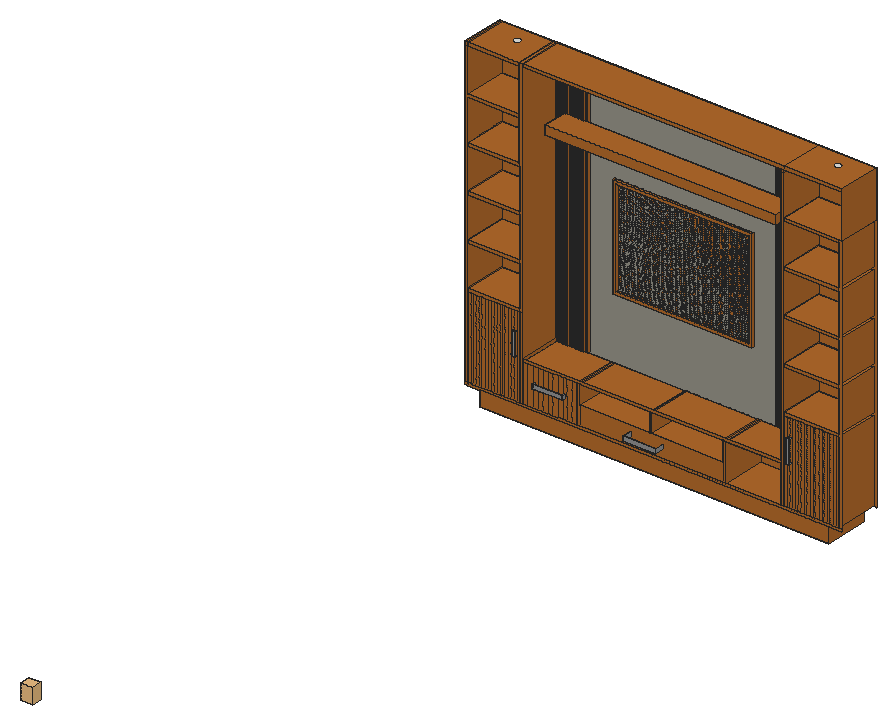
# SketchUp Ruby script. Lengths in millimetres.
U = 1.mm
M = Sketchup.active_model
def pt(a) = Geom::Point3d.new(a.map { |v| v * U })
def face(e, loops, mat)
  f = e.add_face(loops[0].map { |a| pt(a) })
  loops[1..].each { |l| e.add_face(l.map { |a| pt(a) }).erase! }
  f.material = f.back_material = mat if mat
  f
end
# faces: each face lists its corners as indices into pts; further lists are holes
def faces(e, pts, list, mat = nil) = list.each { |f| face(e, (f[0].is_a?(Array) ? f : [f]).map { |l| l.map { |i| pts[i] } }, mat) }
# xy, xz, yz: faces in a plane at the given z, y or x. An outline is a flat list of corners, or four numbers for a rectangle; further outlines are holes
def ring(l) = l.size == 4 ? [[l[0], l[1]], [l[2], l[1]], [l[2], l[3]], [l[0], l[3]]] : l.each_slice(2).to_a
def flat(e, list, mat, &to3) = list.each { |f| face(e, (f[0].is_a?(Array) ? f : [f]).map { |l| ring(l).map { |u, v| to3.(u, v) } }, mat) }
def xy(e, z, list, mat = nil) = flat(e, list, mat) { |x, y| [x, y, z] }
def xz(e, y, list, mat = nil) = flat(e, list, mat) { |x, z| [x, y, z] }
def yz(e, x, list, mat = nil) = flat(e, list, mat) { |y, z| [x, y, z] }
def lines(e, pts, list) = list.each { |a, b| e.add_line(pt(pts[a]), pt(pts[b])) }
# prism: a flat outline (further loops are holes) pulled along v
def prism(e, loops, v, mat = nil)
  f = face(e, loops, mat); d = Geom::Vector3d.new(v.map { |x| x * U })
  f.pushpull(f.normal.samedirection?(d) ? d.length : -d.length)
end
def box(e, o, s, mat = nil) = prism(e, [[o, [o[0] + s[0], o[1], o[2]], [o[0] + s[0], o[1] + s[1], o[2]], [o[0], o[1] + s[1], o[2]]]], [0, 0, s[2]], mat)
def at(x, y, z, deg = 0) = Geom::Transformation.translation(pt([x, y, z])) * Geom::Transformation.rotation(ORIGIN, Z_AXIS, deg.degrees)
def axes(o, x, y, z) = Geom::Transformation.new([*x, 0, *y, 0, *z, 0, *pt(o).to_a, 1])
def part(name) = M.definitions.add(name)
# library, detail: a bought-in or finely detailed component or shape, given as its bounding box
def library(name, o, s) = part(name).tap { |d| box(d.entities, o, s) }
def detail(e, o, s) = box(e.add_group.entities, o, s)
def put(e, d, t, mat = nil) = e.add_instance(d, t).tap { |i| i.material = mat if mat }
def group(e, t, mat = nil) = e.add_group.tap { |g| g.transformation = t; g.material = mat if mat }.entities
root = M.entities
M.materials.add("[Formica Graystone]").color = [149, 146, 135]
M.materials.add("[Metal Embossed]").color = [144, 144, 144]
M.materials.add("[Metal Rough]").color = [153, 157, 160]
M.materials.add("[Wood Bamboo]").color = [177, 105, 43]
c1 = library("Group145\#1",[149.2,164.2,242.8],[528.4,257.1,288.5])
xy(root,2329.8,[[2393.4,174.9,2398.1,175.5,2402.4,177.3,2406.2,180.1,2409,183.9,2410.8,188.2,2411.4,192.9,2410.8,197.5,2409,201.9,2406.2,205.6,2402.4,208.5,2398.1,210.3,2393.4,210.9,2388.8,210.3,2384.4,208.5,2380.7,205.6,2377.8,201.9,2376,197.5,2375.4,192.9,2376,188.2,2377.8,183.9,2380.7,180.1,2384.4,177.3,2388.8,175.5],[246.3,208.1,251.5,208.8,256.3,210.8,260.5,213.9,263.7,218.1,265.7,222.9,266.4,228.1,265.7,233.2,263.7,238.1,260.6,242.2,256.5,245.4,251.6,247.4,246.5,248.1,241.3,247.5,236.5,245.5,232.3,242.3,229.1,238.2,227.1,233.4,226.4,228.2,227,223,229,218.2,232.2,214.1,236.3,210.9,241.1,208.8]])
xy(root,2629.8,[[231.5,187.1,236.1,187.7,240.5,189.5,244.2,192.3,247.1,196.1,248.9,200.4,249.5,205.1,248.9,209.7,247.1,214.1,244.2,217.8,240.5,220.6,236.1,222.4,231.5,223.1,226.8,222.4,222.5,220.6,218.7,217.8,215.9,214.1,214.1,209.7,213.5,205.1,214.1,200.4,215.9,196.1,218.7,192.3,222.5,189.5,226.8,187.7],[2395.6,206.5,2400.2,206.8,2404.7,208.2,2408.7,210.7,2411.8,214.2,2414,218.4,2415,223,2414.8,227.7,2413.3,232.1,2410.8,236.1,2407.3,239.3,2403.1,241.4,2398.5,242.4,2393.9,242.2,2389.4,240.7,2385.4,238.2,2382.3,234.7,2380.1,230.6,2379.1,226,2379.3,221.3,2380.8,216.8,2383.3,212.8,2386.8,209.7,2391,207.5]])
xy(root,2929.8,[[244.8,192,249.5,192.4,253.9,193.9,257.8,196.6,260.9,200.1,262.9,204.4,263.8,209,263.4,213.7,261.9,218.1,259.2,222,255.7,225,251.4,227.1,246.8,228,242.1,227.6,237.7,226.1,233.8,223.4,230.8,219.8,228.7,215.6,227.8,211,228.2,206.3,229.7,201.9,232.4,198,236,194.9,240.2,192.9],[2398.3,207.7,2403,208.3,2407.3,210.1,2411.1,213,2413.9,216.7,2415.7,221,2416.3,225.7,2415.7,230.4,2413.9,234.7,2411.1,238.4,2407.3,241.3,2403,243.1,2398.3,243.7,2393.7,243.1,2389.3,241.3,2385.6,238.4,2382.8,234.7,2381,230.4,2380.3,225.7,2381,221,2382.8,216.7,2385.6,213,2389.3,210.1,2393.7,208.3]])
xy(root,3118.8,[[1326.6,220.4,1331.8,221.1,1336.6,223.1,1340.8,226.3,1344,230.4,1346,235.2,1346.6,240.4,1346,245.6,1344,250.4,1340.8,254.6,1336.6,257.7,1331.8,259.7,1326.6,260.4,1321.5,259.7,1316.6,257.7,1312.5,254.6,1309.3,250.4,1307.3,245.6,1306.6,240.4,1307.3,235.2,1309.3,230.4,1312.5,226.3,1316.6,223.1,1321.5,221.1],[779,222.1,784.2,222.8,789,224.8,793.1,228,796.3,232.1,798.3,236.9,799,242.1,798.3,247.3,796.3,252.1,793.1,256.3,789,259.4,784.2,261.4,779,262.1,773.8,261.4,769,259.4,764.8,256.3,761.7,252.1,759.7,247.3,759,242.1,759.7,236.9,761.7,232.1,764.8,228,769,224.8,773.8,222.8],[1912.4,226.4,1917.6,227.1,1922.4,229.1,1926.6,232.3,1929.7,236.4,1931.7,241.2,1932.4,246.4,1931.7,251.6,1929.7,256.4,1926.6,260.6,1922.4,263.7,1917.6,265.7,1912.4,266.4,1907.2,265.7,1902.4,263.7,1898.3,260.6,1895.1,256.4,1893.1,251.6,1892.4,246.4,1893.1,241.2,1895.1,236.4,1898.3,232.3,1902.4,229.1,1907.2,227.1]])
xy(root,3229.8,[[223.6,166.8,228.3,167.4,232.6,169.2,236.3,172.1,239.2,175.8,241,180.2,241.6,184.8,241,189.5,239.2,193.8,236.3,197.5,232.6,200.4,228.3,202.2,223.6,202.8,219,202.2,214.6,200.4,210.9,197.5,208,193.8,206.2,189.5,205.6,184.8,206.2,180.2,208,175.8,210.9,172.1,214.6,169.2,219,167.4],[2406.8,198.3,2411.5,198.9,2415.8,200.7,2419.5,203.6,2422.4,207.3,2424.2,211.7,2424.8,216.3,2424.2,221,2422.4,225.3,2419.5,229,2415.8,231.9,2411.5,233.7,2406.8,234.3,2402.2,233.7,2397.8,231.9,2394.1,229,2391.2,225.3,2389.4,221,2388.8,216.3,2389.4,211.7,2391.2,207.3,2394.1,203.6,2397.8,200.7,2402.2,198.9]])
xy(root,3549.8,[[572.3,169.1,577.5,169.8,582.3,171.8,586.4,174.9,589.6,179.1,591.6,183.9,592.3,189.1,591.6,194.3,589.6,199.1,586.4,203.2,582.3,206.4,577.5,208.4,572.3,209.1,567.1,208.4,562.3,206.4,558.1,203.2,555,199.1,553,194.3,552.3,189.1,553,183.9,555,179.1,558.1,174.9,562.3,171.8,567.1,169.8],[1994,197.3,1999.2,198,2004,200,2008.2,203.1,2011.3,207.3,2013.3,212.1,2014,217.3,2013.3,222.5,2011.3,227.3,2008.2,231.4,2004,234.6,1999.2,236.6,1994,237.3,1988.8,236.6,1984,234.6,1979.9,231.4,1976.7,227.3,1974.7,222.5,1974,217.3,1974.7,212.1,1976.7,207.3,1979.9,203.1,1984,200,1988.8,198],[1316,214,1321.2,214.7,1326,216.7,1330.1,219.9,1333.3,224,1335.3,228.9,1336,234,1335.3,239.2,1333.3,244,1330.1,248.2,1326,251.4,1321.2,253.4,1316,254,1310.8,253.4,1306,251.4,1301.8,248.2,1298.7,244,1296.7,239.2,1296,234,1296.7,228.9,1298.7,224,1301.8,219.9,1306,216.7,1310.8,214.7]])
xy(root,3569.8,[[215.9,228.9,220.6,229.6,224.9,231.4,228.7,234.2,231.5,237.9,233.3,242.3,233.9,246.9,233.3,251.6,231.5,255.9,228.7,259.7,224.9,262.5,220.6,264.3,215.9,264.9,211.3,264.3,206.9,262.5,203.2,259.7,200.4,255.9,198.6,251.6,197.9,246.9,198.6,242.3,200.4,237.9,203.2,234.2,206.9,231.4,211.3,229.6],[2424.7,232.7,2429.4,233.4,2433.7,235.2,2437.5,238,2440.3,241.7,2442.1,246.1,2442.7,250.7,2442.1,255.4,2440.3,259.7,2437.5,263.5,2433.7,266.3,2429.4,268.1,2424.7,268.7,2420.1,268.1,2415.7,266.3,2412,263.5,2409.1,259.7,2407.3,255.4,2406.7,250.7,2407.3,246.1,2409.1,241.7,2412,238,2415.7,235.2,2420.1,233.4]])
xz(root,62,[[105,1349.8,2515,1449.8],[20,1469.8,40,2029.8],[40,1469.8,60,2029.8],[60,1469.8,80,2029.8],[80,1469.8,100,2029.8],
  [100,1469.8,120,2029.8],[120,1469.8,140,2029.8],[140,1469.8,160,2029.8],[160,1469.8,180,2029.8],[180,1469.8,200,2029.8],
  [200,1469.8,220,2029.8],[220,1469.8,240,2029.8],[240,1469.8,260,2029.8],[260,1469.8,280,2029.8],[280,1469.8,300,2029.8],
  [300,1469.8,320,2029.8],[320,1469.8,340,2029.8],[340,1469.8,360,2029.8],[360,1469.8,380,2029.8],[380,1469.8,400,2029.8],
  [400,1469.8,436.1,1729.8],[436.1,1469.8,470.1,1729.8],[470.1,1469.8,504.1,1729.8],[504.1,1469.8,538.1,1729.8],[538.1,1469.8,572.1,1729.8],
  [572.1,1469.8,606.1,1729.8],[606.1,1469.8,640.1,1729.8],[640.1,1469.8,674.1,1729.8],[674.1,1469.8,708.1,1729.8],[708.1,1469.8,742.1,1729.8],
  [742.1,1469.8,776.2,1729.8],[2200,1469.8,2220,2029.8],[2220,1469.8,2240,2029.8],[2240,1469.8,2260,2029.8],[2260,1469.8,2280,2029.8],
  [2280,1469.8,2299,2029.8],[2299,1469.8,2319,2029.8],[2319,1469.8,2339,2029.8],[2339,1469.8,2359,2029.8],[2359,1469.8,2379,2029.8],
  [2379,1469.8,2399,2029.8],[2399,1469.8,2419,2029.8],[2419,1469.8,2440,2029.8],[2440,1469.8,2461,2029.8],[2461,1469.8,2481,2029.8],
  [2481,1469.8,2501,2029.8],[2501,1469.8,2521,2029.8],[2521,1469.8,2541,2029.8],[2541,1469.8,2561,2029.8],[2561,1469.8,2580,2029.8]],"[Wood Bamboo]")
xz(root,362,[[[798.5,2166.1,1754.5,2871.1],[818.5,2186.1,1734.5,2851.1]]])
p = [[380,62,2049.8],[380,62,2029.8],[2100,362,3529.8],[2100,365,3529.8],[20,62,3549.8],[20,62,3569.8],
  [0,62,3569.8],[0,62,3549.8],[2180,362,1749.8],[2180,362,1729.8],[2198,362,3569.8],[2198,362,3529.8],
  [2198,362,1729.8],[2198,362,1749.8],[414,362,3569.8],[412,362,1729.8],[394,344,1749.8],[414,344,1749.8],
  [394,362,1749.8],[414,362,1749.8],[483.9,59,1629.2],[483.9,62,1629.2],[686,59,1629.2],[686,62,1629.2]]
lines(root,p,[[0,1],[2,3],[4,5],[5,6],[6,7],[8,9],[10,11],[12,9],[13,12],[11,13],[14,10],[9,15],
  [16,17],[18,16],[19,17],[20,21],[22,23]])
put(root,c1,axes([3219.9,-7703.5,4008.9],[0.15946,0,0],[0,-0.2848,0],[0,0,0.37371]))
g1 = group(root,at(0,62,1349.8),"[Wood Bamboo]")
xy(g1,0,[[105,0,2515,300]],"[Wood Bamboo]")
xy(g1,100,[[105,0,2515,300]],"[Wood Bamboo]")
xy(g1,120,[[0,0,20,300],[20,0,380,300],[380,0,400,300],[400,0,776.2,300],[776.2,0,1804,300],
  [1804,0,2180,300],[2180,0,2200,300],[2200,0,2580,300]],"[Wood Bamboo]")
xy(g1,179,[[1143,-62,1143,0,1148.5,0,1148.5,-56.4,1364.4,-56.4,1364.4,0,1370,0,1370,-62]],"[Metal Embossed]")
xy(g1,207,[[1143,-62,1370,-62,1370,0,1364.4,0,1364.4,-56.4,1148.5,-56.4,1148.5,0,1143,0]],"[Metal Embossed]")
xy(g1,250,[[796.2,0,1280.1,300],[1290.1,0,1784,300]],"[Wood Bamboo]")
xy(g1,251.4,[[481,-18,481,0,483.9,0,483.9,-15,686,-15,686,0,689,0,689,-18]],"[Metal Embossed]")
xy(g1,279.4,[[481,-18,689,-18,689,0,686,0,686,-15,483.9,-15,483.9,0,481,0]],"[Metal Embossed]")
xy(g1,380,[[400,0,776.2,300],[776.2,0,796.2,300],[796.2,0,1280.1,300],[1280.1,0,1290.1,300],[1290.1,0,1784,300],
  [1784,0,1804,300],[1804,0,2180,300]],"[Wood Bamboo]")
xy(g1,400,[[340,-18,360,0],[2228.7,-18,2248.7,0]])
xy(g1,400,[[422.1,264.2,436.1,282.2],[444.1,264.4,458.1,282.4],[466.2,264.7,480.2,282.7],[488.3,264.9,502.3,282.9],[510.4,265.1,524.4,283.1],
  [532.4,265.3,546.4,283.3],[554.5,265.6,568.5,283.6],[576.6,265.8,590.6,283.8],[598.7,266,612.7,284],[620.7,266.2,634.7,284.2],
  [1923.2,279.5,1937.2,297.5],[1945.3,279.7,1959.3,297.7],[1967.3,280,1981.3,298],[1989.4,280.2,2003.4,298.2],[2011.5,280.4,2025.5,298.4],
  [2033.6,280.6,2047.6,298.6],[2055.6,280.9,2069.6,298.9],[2077.7,281.1,2091.7,299.1],[2099.8,281.3,2113.8,299.3],[2121.9,281.5,2135.9,299.5],
  [2143.9,281.8,2157.9,299.8],[394,282,400,300],[400,282,414,300]],"[Wood Bamboo]")
xy(g1,402.5,[[340,-15.5,360,0],[2228.7,-15.5,2248.7,0]],"[Metal Rough]")
xy(g1,555,[[340,-15.5,360,0],[2228.7,-15.5,2248.7,0]],"[Metal Rough]")
xy(g1,557.5,[[340,-18,360,0],[2228.7,-18,2248.7,0]],"[Metal Rough]")
xy(g1,680,[[20,0,380,300],[2200,0,2580,300]],"[Wood Bamboo]")
xy(g1,700,[[20,0,380,300],[2200,0,2580,300]],"[Wood Bamboo]")
xy(g1,816.3,[[798.5,282,1754.5,300]])
xy(g1,836.3,[[818.5,282,1734.5,300]])
xy(g1,980,[[20,0,380,300],[2200,0,2580,300]],"[Wood Bamboo]")
xy(g1,1000,[[20,0,380,300],[2200,0,2580,300]],"[Wood Bamboo]")
xy(g1,1280,[[20,0,380,300],[2200,0,2580,300]],"[Wood Bamboo]")
xy(g1,1300,[[20,0,380,300],[2200,0,2580,300]],"[Wood Bamboo]")
xy(g1,1501.3,[[818.5,282,1734.5,300]])
xy(g1,1521.3,[[798.5,282,1754.5,300]])
xy(g1,1580,[[20,0,380,300],[2200,0,2580,300]],"[Wood Bamboo]")
xy(g1,1600,[[20,0,374,300],[2200,0,2580,300]],"[Wood Bamboo]")
xy(g1,1769,[[480.2,94.7,2069.6,264.7]],"[Wood Bamboo]")
xy(g1,1831.5,[[480.2,94.7,2069.6,264.7]],"[Wood Bamboo]")
xy(g1,1880,[[20,0,374,251.5],[2200,0,2580,300],[20,251.5,374,300]],"[Wood Bamboo]")
xy(g1,1900,[[20,0,374,300],[2200,0,2600,300]],"[Wood Bamboo]")
xy(g1,2200,[[[400,0,2180,0,2180,282,2166,282,2166,300,414,300,414,282,400,282],[2077.7,281.1,2091.7,299.1],[2121.9,281.5,2135.9,299.5],[598.7,266,612.7,284],[1923.2,279.5,1937.2,297.5],[1967.3,280,1981.3,298],[576.6,265.8,590.6,283.8],[1945.3,279.7,1959.3,297.7],[422.1,264.2,436.1,282.2],[444.1,264.4,458.1,282.4],[466.2,264.7,480.2,282.7],[488.3,264.9,502.3,282.9],[510.4,265.1,524.4,283.1],[532.4,265.3,546.4,283.3],[554.5,265.6,568.5,283.6],[620.7,266.2,634.7,284.2],[1989.4,280.2,2003.4,298.2],[2011.5,280.4,2025.5,298.4],[2033.6,280.6,2047.6,298.6],[2055.6,280.9,2069.6,298.9],[2099.8,281.3,2113.8,299.3],[2143.9,281.8,2157.9,299.8]],[2180,0,2200,300],[422.1,264.2,436.1,282.2],[444.1,264.4,458.1,282.4],[466.2,264.7,480.2,282.7],
  [488.3,264.9,502.3,282.9],[510.4,265.1,524.4,283.1],[532.4,265.3,546.4,283.3],[554.5,265.6,568.5,283.6],[576.6,265.8,590.6,283.8],
  [598.7,266,612.7,284],[620.7,266.2,634.7,284.2],[1923.2,279.5,1937.2,297.5],[1945.3,279.7,1959.3,297.7],[1967.3,280,1981.3,298],
  [1989.4,280.2,2003.4,298.2],[2011.5,280.4,2025.5,298.4],[2033.6,280.6,2047.6,298.6],[2055.6,280.9,2069.6,298.9],[2077.7,281.1,2091.7,299.1],
  [2099.8,281.3,2113.8,299.3],[2121.9,281.5,2135.9,299.5],[2143.9,281.8,2157.9,299.8],[394,282,414,300],[2166,282,2180,300]],"[Wood Bamboo]")
xy(g1,2220,[[0,0,20,300],[20,0,374,300],[374,0,400,0,400,282,394,282,394,300,374,300],[400,0,2200,0,2200,300,394,300,394,282,400,282],[2200,0,2600,300]],"[Wood Bamboo]")
xz(g1,-62,[[1143,179,1370,207]],"[Metal Embossed]")
xz(g1,-56.4,[[1148.5,179,1364.4,207]],"[Wood Bamboo]")
xz(g1,-18,[[481,251.4,689,279.4]],"[Metal Embossed]")
xz(g1,-18,[[340,400,360,557.5],[2228.7,400,2248.7,557.5]],"[Metal Rough]")
xz(g1,-15.5,[[340,402.5,360,555],[2228.7,402.5,2248.7,555]],"[Metal Rough]")
xz(g1,-15,[[483.9,251.4,686,279.4]])
xz(g1,0,[[481,251.4,483.9,279.4],[686,251.4,689,279.4],[340,400,360,402.5],[2228.7,400,2248.7,402.5],[340,555,360,557.5],
  [2228.7,555,2248.7,557.5]])
xz(g1,0,[[340,402.5,360,555],[2228.7,402.5,2248.7,555]],"[Metal Rough]")
xz(g1,0,[[0,100,20,120],[20,100,2600,120],[0,120,20,120,20,1880,374,1880,374,1900,20,1900,20,2200,0,2200],[380,120,400,120,400,2220,374,2220,374,1600,380,1600],[776.2,120,796.2,380],
  [[796.2,120,1784,250],[1364.4,179,1370,207],[1143,179,1148.5,207]],[1784,120,1804,380],[2180,120,2200,2180],[2580,120,2600,1900],[1280.1,250,1290.1,380],
  [400,380,2180,400],[20,680,380,700],[2200,680,2580,700],[20,980,380,1000],[2200,980,2580,1000],
  [20,1280,380,1300],[2200,1280,2580,1300],[20,1580,380,1600],[2200,1580,2580,1600],[2200,1880,2580,1900],
  [2180,2180,2200,2200],[0,2200,20,2220],[20,2200,374,2220],[400,2200,2200,2220],[2200,2200,2600,2220]],"[Wood Bamboo]")
xz(g1,94.7,[[480.2,1769,2069.6,1831.5]],"[Wood Bamboo]")
xz(g1,264.2,[[422.1,400,436.1,2200]],"[Wood Bamboo]")
xz(g1,264.4,[[444.1,400,458.1,2200]],"[Wood Bamboo]")
xz(g1,264.7,[[466.2,400,480.2,2200],[480.2,1769,2069.6,1831.5]],"[Wood Bamboo]")
xz(g1,264.9,[[488.3,400,502.3,2200]],"[Wood Bamboo]")
xz(g1,265.1,[[510.4,400,524.4,2200]],"[Wood Bamboo]")
xz(g1,265.3,[[532.4,400,546.4,2200]],"[Wood Bamboo]")
xz(g1,265.6,[[554.5,400,568.5,2200]],"[Wood Bamboo]")
xz(g1,265.8,[[576.6,400,590.6,2200]],"[Wood Bamboo]")
xz(g1,266,[[598.7,400,612.7,2200]],"[Wood Bamboo]")
xz(g1,266.2,[[620.7,400,634.7,2200]],"[Wood Bamboo]")
xz(g1,279.5,[[1923.2,400,1937.2,2200]],"[Wood Bamboo]")
xz(g1,279.7,[[1945.3,400,1959.3,2200]],"[Wood Bamboo]")
xz(g1,280,[[1967.3,400,1981.3,2200]],"[Wood Bamboo]")
xz(g1,280.2,[[1989.4,400,2003.4,2200]],"[Wood Bamboo]")
xz(g1,280.4,[[2011.5,400,2025.5,2200]],"[Wood Bamboo]")
xz(g1,280.6,[[2033.6,400,2047.6,2200]],"[Wood Bamboo]")
xz(g1,280.9,[[2055.6,400,2069.6,2200]],"[Wood Bamboo]")
xz(g1,281.1,[[2077.7,400,2091.7,2200]],"[Wood Bamboo]")
xz(g1,281.3,[[2099.8,400,2113.8,2200]],"[Wood Bamboo]")
xz(g1,281.5,[[2121.9,400,2135.9,2200]],"[Wood Bamboo]")
xz(g1,281.8,[[2143.9,400,2157.9,2200]],"[Wood Bamboo]")
xz(g1,282,[[[798.5,816.3,1754.5,1521.3],[818.5,836.3,1734.5,1501.3]]])
xz(g1,282,[[394,400,400,2200],[2166,400,2180,2200],[394,2200,400,2220]],"[Wood Bamboo]")
xz(g1,282.2,[[422.1,400,436.1,2200]],"[Wood Bamboo]")
xz(g1,282.4,[[444.1,400,458.1,2200]],"[Wood Bamboo]")
xz(g1,282.7,[[466.2,400,480.2,2200]],"[Wood Bamboo]")
xz(g1,282.9,[[488.3,400,502.3,2200]],"[Wood Bamboo]")
xz(g1,283.1,[[510.4,400,524.4,2200]],"[Wood Bamboo]")
xz(g1,283.3,[[532.4,400,546.4,2200]],"[Wood Bamboo]")
xz(g1,283.6,[[554.5,400,568.5,2200]],"[Wood Bamboo]")
xz(g1,283.8,[[576.6,400,590.6,2200]],"[Wood Bamboo]")
xz(g1,284,[[598.7,400,612.7,2200]],"[Wood Bamboo]")
xz(g1,284.2,[[620.7,400,634.7,2200]],"[Wood Bamboo]")
xz(g1,297.5,[[1923.2,400,1937.2,2200]],"[Wood Bamboo]")
xz(g1,297.7,[[1945.3,400,1959.3,2200]],"[Wood Bamboo]")
xz(g1,298,[[1967.3,400,1981.3,2200]],"[Wood Bamboo]")
xz(g1,298.2,[[1989.4,400,2003.4,2200]],"[Wood Bamboo]")
xz(g1,298.4,[[2011.5,400,2025.5,2200]],"[Wood Bamboo]")
xz(g1,298.6,[[2033.6,400,2047.6,2200]],"[Wood Bamboo]")
xz(g1,298.9,[[2055.6,400,2069.6,2200]],"[Wood Bamboo]")
xz(g1,299.1,[[2077.7,400,2091.7,2200]],"[Wood Bamboo]")
xz(g1,299.3,[[2099.8,400,2113.8,2200]],"[Wood Bamboo]")
xz(g1,299.5,[[2121.9,400,2135.9,2200]],"[Wood Bamboo]")
xz(g1,299.8,[[2143.9,400,2157.9,2200]],"[Wood Bamboo]")
xz(g1,300,[[[798.5,816.3,1754.5,1521.3],[818.5,836.3,1734.5,1501.3]],[818.5,836.3,1734.5,1501.3]])
xz(g1,300,[[105,0,2515,100],[0,120,20,2220],[20,120,374,680],[374,120,380,680],[380,120,400,120,400,400,394,400,394,2220,374,2220,374,1580,380,1580,380,1300,374,1300,374,1280,380,1280,380,1000,374,1000,374,980,380,980,380,700,374,700,374,680,380,680],
  [400,120,776.2,380],[776.2,120,1804,120,1804,380,1784,380,1784,250,1290.1,250,1290.1,380,1280.1,380,1280.1,250,796.2,250,796.2,380,776.2,380],[1804,120,2180,380],[2180,120,2200,380],[2200,120,2580,680],
  [2580,120,2600,120,2600,1900,2200,1900,2200,1880,2580,1880,2580,1600,2200,1600,2200,1580,2580,1580,2580,1300,2200,1300,2200,1280,2580,1280,2580,1000,2200,1000,2200,980,2580,980,2580,700,2200,700,2200,680,2580,680],[796.2,250,1280.1,380],[1290.1,250,1784,380],[394,400,400,2200],[20,680,374,700],
  [20,700,374,980],[374,700,380,980],[2200,700,2580,980],[20,980,374,1000],[20,1000,374,1280],
  [374,1000,380,1280],[2200,1000,2580,1280],[20,1280,374,1300],[20,1300,374,1580],[374,1300,380,1580],
  [2200,1300,2580,1580],[20,1580,374,1600],[20,1600,374,1880],[2200,1600,2580,1880],[20,1880,374,1900],
  [20,1900,374,2220],[2200,1900,2600,2220],[394,2200,2200,2220]],"[Wood Bamboo]")
yz(g1,0,[[0,120,300,2220]],"[Wood Bamboo]")
yz(g1,20,[[0,120,300,680],[0,680,300,700],[0,700,300,980],[0,980,300,1000],[0,1000,300,1280],
  [0,1280,300,1300],[0,1300,300,1580],[0,1580,300,1600],[0,1600,300,1880],[0,1900,300,2220]],"[Wood Bamboo]")
yz(g1,105,[[0,0,300,100]],"[Wood Bamboo]")
yz(g1,340,[[-18,400,-18,557.5,0,557.5,0,555,-15.5,555,-15.5,402.5,0,402.5,0,400]],"[Metal Rough]")
yz(g1,360,[[-18,400,0,400,0,402.5,-15.5,402.5,-15.5,555,0,555,0,557.5,-18,557.5]],"[Metal Rough]")
yz(g1,374,[[0,1600,300,1880],[0,1880,300,1900],[0,1900,300,2220]],"[Wood Bamboo]")
yz(g1,380,[[0,120,300,680],[0,700,300,980],[0,1000,300,1280],[0,1300,300,1580]],"[Wood Bamboo]")
yz(g1,394,[[282,400,300,2200],[282,2200,300,2220]],"[Wood Bamboo]")
yz(g1,400,[[0,120,300,380],[0,380,300,400],[0,400,282,2200],[0,2200,282,2220]],"[Wood Bamboo]")
yz(g1,422.1,[[264.2,400,282.2,2200]],"[Wood Bamboo]")
yz(g1,436.1,[[264.2,400,282.2,2200]],"[Wood Bamboo]")
yz(g1,444.1,[[264.4,400,282.4,2200]],"[Wood Bamboo]")
yz(g1,458.1,[[264.4,400,282.4,2200]],"[Wood Bamboo]")
yz(g1,466.2,[[264.7,400,282.7,2200]],"[Wood Bamboo]")
yz(g1,480.2,[[264.7,400,282.7,2200],[94.7,1769,264.7,1831.5]],"[Wood Bamboo]")
yz(g1,481,[[-18,251.4,0,279.4]],"[Metal Embossed]")
yz(g1,483.9,[[-15,251.4,0,279.4]],"[Metal Embossed]")
yz(g1,488.3,[[264.9,400,282.9,2200]],"[Wood Bamboo]")
yz(g1,502.3,[[264.9,400,282.9,2200]],"[Wood Bamboo]")
yz(g1,510.4,[[265.1,400,283.1,2200]],"[Wood Bamboo]")
yz(g1,524.4,[[265.1,400,283.1,2200]],"[Wood Bamboo]")
yz(g1,532.4,[[265.3,400,283.3,2200]],"[Wood Bamboo]")
yz(g1,546.4,[[265.3,400,283.3,2200]],"[Wood Bamboo]")
yz(g1,554.5,[[265.6,400,283.6,2200]],"[Wood Bamboo]")
yz(g1,568.5,[[265.6,400,283.6,2200]],"[Wood Bamboo]")
yz(g1,576.6,[[265.8,400,283.8,2200]],"[Wood Bamboo]")
yz(g1,590.6,[[265.8,400,283.8,2200]],"[Wood Bamboo]")
yz(g1,598.7,[[266,400,284,2200]],"[Wood Bamboo]")
yz(g1,612.7,[[266,400,284,2200]],"[Wood Bamboo]")
yz(g1,620.7,[[266.2,400,284.2,2200]],"[Wood Bamboo]")
yz(g1,634.7,[[266.2,400,284.2,2200]],"[Wood Bamboo]")
yz(g1,686,[[-15,251.4,0,279.4]],"[Metal Embossed]")
yz(g1,689,[[-18,251.4,0,279.4]],"[Metal Embossed]")
yz(g1,776.2,[[0,120,300,380]],"[Wood Bamboo]")
yz(g1,796.2,[[0,250,300,380]],"[Wood Bamboo]")
yz(g1,798.5,[[282,816.3,300,1521.3]])
yz(g1,818.5,[[282,836.3,300,1501.3]])
yz(g1,1143,[[-62,179,0,207]],"[Metal Embossed]")
yz(g1,1148.5,[[-56.4,179,0,207]],"[Metal Embossed]")
yz(g1,1280.1,[[0,250,300,380]],"[Wood Bamboo]")
yz(g1,1290.1,[[0,250,300,380]],"[Wood Bamboo]")
yz(g1,1364.4,[[-56.4,179,0,207]],"[Wood Bamboo]")
yz(g1,1370,[[-62,179,0,207]],"[Metal Embossed]")
yz(g1,1734.5,[[282,836.3,300,1501.3]])
yz(g1,1754.5,[[282,816.3,300,1521.3]])
yz(g1,1784,[[0,250,300,380]],"[Wood Bamboo]")
yz(g1,1804,[[0,120,300,380]],"[Wood Bamboo]")
yz(g1,1923.2,[[279.5,400,297.5,2200]],"[Wood Bamboo]")
yz(g1,1937.2,[[279.5,400,297.5,2200]],"[Wood Bamboo]")
yz(g1,1945.3,[[279.7,400,297.7,2200]],"[Wood Bamboo]")
yz(g1,1959.3,[[279.7,400,297.7,2200]],"[Wood Bamboo]")
yz(g1,1967.3,[[280,400,298,2200]],"[Wood Bamboo]")
yz(g1,1981.3,[[280,400,298,2200]],"[Wood Bamboo]")
yz(g1,1989.4,[[280.2,400,298.2,2200]],"[Wood Bamboo]")
yz(g1,2003.4,[[280.2,400,298.2,2200]],"[Wood Bamboo]")
yz(g1,2011.5,[[280.4,400,298.4,2200]],"[Wood Bamboo]")
yz(g1,2025.5,[[280.4,400,298.4,2200]],"[Wood Bamboo]")
yz(g1,2033.6,[[280.6,400,298.6,2200]],"[Wood Bamboo]")
yz(g1,2047.6,[[280.6,400,298.6,2200]],"[Wood Bamboo]")
yz(g1,2055.6,[[280.9,400,298.9,2200]],"[Wood Bamboo]")
yz(g1,2069.6,[[280.9,400,298.9,2200],[94.7,1769,264.7,1831.5]],"[Wood Bamboo]")
yz(g1,2077.7,[[281.1,400,299.1,2200]],"[Wood Bamboo]")
yz(g1,2091.7,[[281.1,400,299.1,2200]],"[Wood Bamboo]")
yz(g1,2099.8,[[281.3,400,299.3,2200]],"[Wood Bamboo]")
yz(g1,2113.8,[[281.3,400,299.3,2200]],"[Wood Bamboo]")
yz(g1,2121.9,[[281.5,400,299.5,2200]],"[Wood Bamboo]")
yz(g1,2135.9,[[281.5,400,299.5,2200]],"[Wood Bamboo]")
yz(g1,2143.9,[[281.8,400,299.8,2200]],"[Wood Bamboo]")
yz(g1,2157.9,[[281.8,400,299.8,2200]],"[Wood Bamboo]")
yz(g1,2180,[[0,120,300,380],[0,400,282,2180],[0,2180,282,2200]],"[Wood Bamboo]")
yz(g1,2200,[[0,120,300,680],[0,680,300,700],[0,700,300,980],[0,980,300,1000],[0,1000,300,1280],
  [0,1280,300,1300],[0,1300,300,1580],[0,1580,300,1600],[0,1600,300,1880],[0,1880,300,1900],
  [0,1900,300,2180],[0,2180,300,2200]],"[Wood Bamboo]")
yz(g1,2228.7,[[-18,400,-18,557.5,0,557.5,0,555,-15.5,555,-15.5,402.5,0,402.5,0,400]],"[Metal Rough]")
yz(g1,2248.7,[[-18,400,0,400,0,402.5,-15.5,402.5,-15.5,555,0,555,0,557.5,-18,557.5]],"[Metal Rough]")
yz(g1,2515,[[0,0,300,100]],"[Wood Bamboo]")
yz(g1,2580,[[0,120,300,680],[0,700,300,980],[0,1000,300,1280],[0,1300,300,1580],[0,1600,300,1880]],"[Wood Bamboo]")
yz(g1,2600,[[0,1900,300,2220]],"[Wood Bamboo]")
p = [[1804,300,120],[1804,300,119],[2166,300,400],[2166,282,400]]
lines(g1,p,[[0,1],[2,3]])
g2 = group(g1,at(400,300,380))
xz(g2,0,[[0,0,1800,1820]],"[Formica Graystone]")
